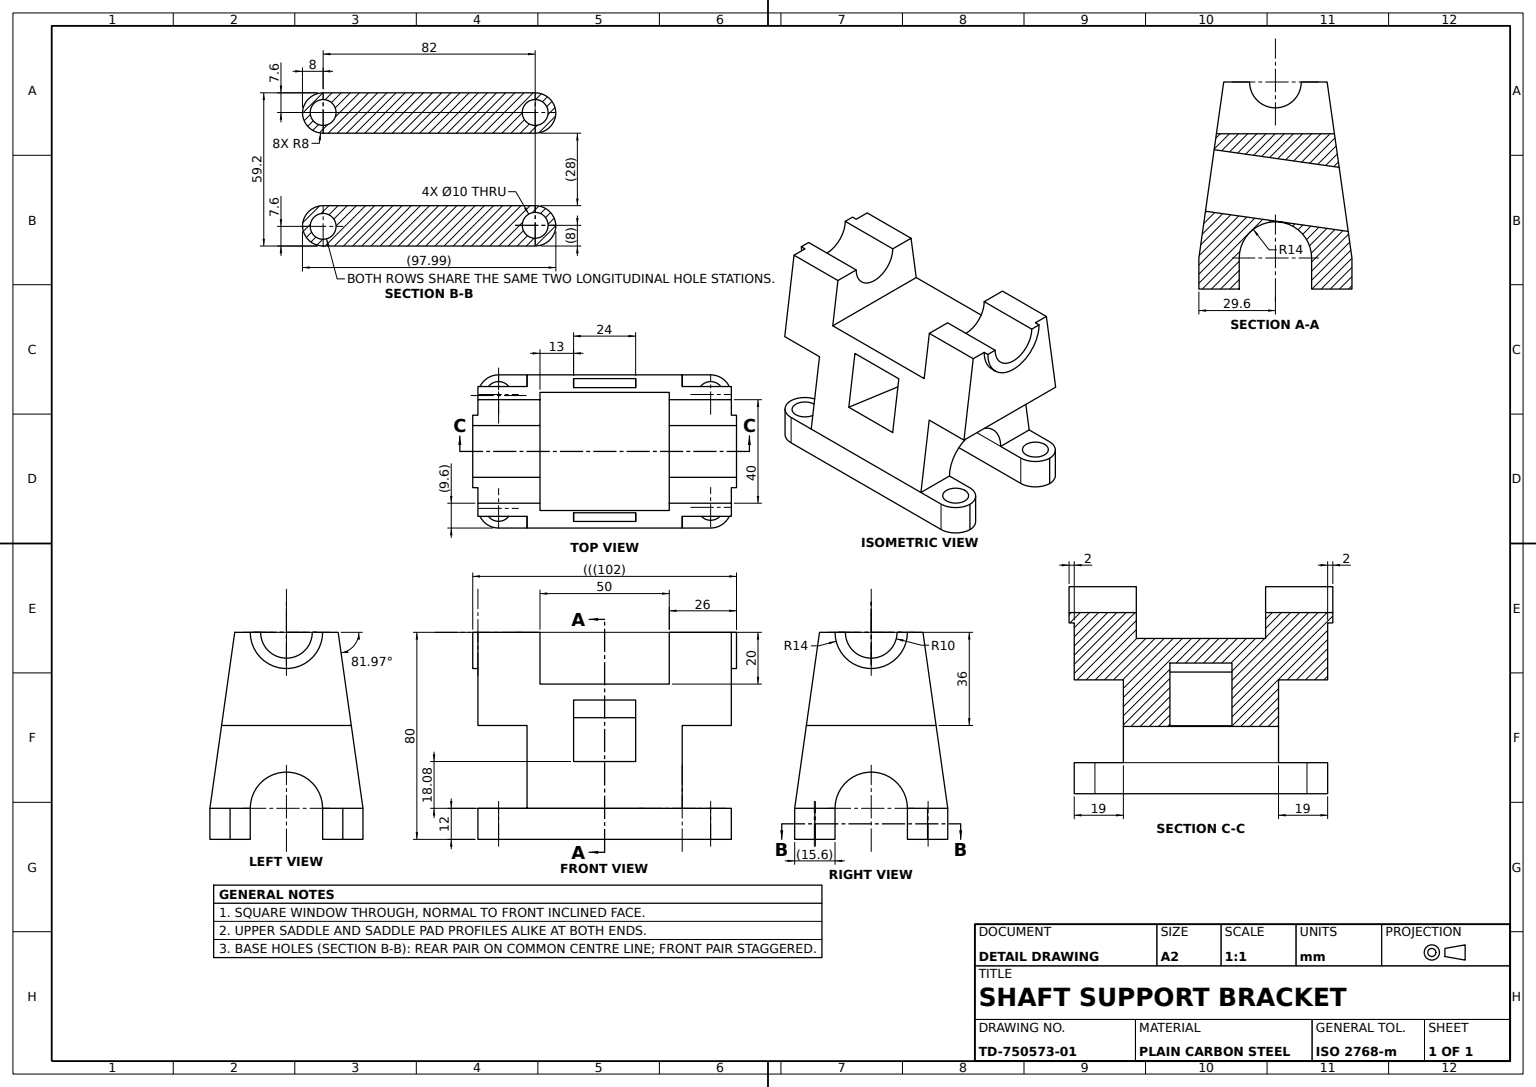
ISO-10303-21;
HEADER;
FILE_DESCRIPTION((''),'2;1');
FILE_NAME('','',(''),(''),'','','');
FILE_SCHEMA(('AUTOMOTIVE_DESIGN'));
ENDSEC;
DATA;
#1=APPLICATION_CONTEXT('');
#2=PRODUCT_CONTEXT('',#1,'mechanical');
#3=PRODUCT('','','',(#2));
#4=PRODUCT_DEFINITION_FORMATION('','',#3);
#5=PRODUCT_DEFINITION_CONTEXT('',#1,'design');
#6=PRODUCT_DEFINITION('','',#4,#5);
#7=PRODUCT_DEFINITION_SHAPE('','',#6);
#8=(LENGTH_UNIT()NAMED_UNIT(*)SI_UNIT(.MILLI.,.METRE.));
#9=(NAMED_UNIT(*)PLANE_ANGLE_UNIT()SI_UNIT($,.RADIAN.));
#10=(NAMED_UNIT(*)SI_UNIT($,.STERADIAN.)SOLID_ANGLE_UNIT());
#11=UNCERTAINTY_MEASURE_WITH_UNIT(LENGTH_MEASURE(1.E-05),#8,'distance_accuracy_value','');
#12=(GEOMETRIC_REPRESENTATION_CONTEXT(3)GLOBAL_UNCERTAINTY_ASSIGNED_CONTEXT((#11))GLOBAL_UNIT_ASSIGNED_CONTEXT((#8,#9,#10))REPRESENTATION_CONTEXT('',''));
#13=CARTESIAN_POINT('',(-49.,80.,-20.));
#14=VERTEX_POINT('',#13);
#15=CARTESIAN_POINT('',(-49.,80.,-14.));
#16=VERTEX_POINT('',#15);
#17=CARTESIAN_POINT('',(-49.,80.,20.));
#18=DIRECTION('',(0.,0.,1.));
#19=VECTOR('',#18,1000.);
#20=LINE('',#17,#19);
#21=EDGE_CURVE('',#14,#16,#20,.T.);
#22=ORIENTED_EDGE('',*,*,#21,.F.);
#23=CARTESIAN_POINT('',(-49.,44.,-25.081638));
#24=VERTEX_POINT('',#23);
#25=CARTESIAN_POINT('',(-49.,12.,-29.598649));
#26=DIRECTION('',(0.,0.990183858,0.139770985));
#27=VECTOR('',#26,1000.);
#28=LINE('',#25,#27);
#29=EDGE_CURVE('',#24,#14,#28,.T.);
#30=ORIENTED_EDGE('',*,*,#29,.F.);
#31=CARTESIAN_POINT('',(-49.,44.,25.081638));
#32=VERTEX_POINT('',#31);
#33=DIRECTION('',(0.,0.,-1.));
#34=VECTOR('',#33,1000.);
#35=LINE('',#23,#34);
#36=EDGE_CURVE('',#32,#24,#35,.T.);
#37=ORIENTED_EDGE('',*,*,#36,.F.);
#38=VERTEX_POINT('',#17);
#39=DIRECTION('',(0.,-0.990183858,0.139770985));
#40=VECTOR('',#39,1000.);
#41=LINE('',#17,#40);
#42=EDGE_CURVE('',#38,#32,#41,.T.);
#43=ORIENTED_EDGE('',*,*,#42,.F.);
#44=CARTESIAN_POINT('',(-49.,80.,14.));
#45=VERTEX_POINT('',#44);
#46=EDGE_CURVE('',#45,#38,#20,.T.);
#47=ORIENTED_EDGE('',*,*,#46,.F.);
#48=CARTESIAN_POINT('',(-49.,80.,0.));
#49=DIRECTION('',(-1.,0.,0.));
#50=AXIS2_PLACEMENT_3D('',#48,#49,#18);
#51=CIRCLE('',#50,14.);
#52=EDGE_CURVE('',#16,#45,#51,.T.);
#53=ORIENTED_EDGE('',*,*,#52,.F.);
#54=EDGE_LOOP('',(#22,#30,#37,#43,#47,#53));
#55=FACE_OUTER_BOUND('',#54,.T.);
#56=CARTESIAN_POINT('',(-49.,12.,29.598649));
#57=DIRECTION('',(1.,0.,0.));
#58=AXIS2_PLACEMENT_3D('',#56,#57,#33);
#59=PLANE('',#58);
#60=ADVANCED_FACE('',(#55),#59,.F.);
#61=CARTESIAN_POINT('',(-41.,0.,17.));
#62=VERTEX_POINT('',#61);
#63=CARTESIAN_POINT('',(-41.,12.,17.));
#64=VERTEX_POINT('',#63);
#65=CARTESIAN_POINT('',(-41.,-8.,17.));
#66=DIRECTION('',(0.,1.,0.));
#67=VECTOR('',#66,1000.);
#68=LINE('',#65,#67);
#69=EDGE_CURVE('',#62,#64,#68,.T.);
#70=ORIENTED_EDGE('',*,*,#69,.F.);
#71=CARTESIAN_POINT('',(-41.,0.,27.));
#72=VERTEX_POINT('',#71);
#73=CARTESIAN_POINT('',(-41.,0.,22.));
#74=DIRECTION('',(0.,-1.,0.));
#75=AXIS2_PLACEMENT_3D('',#73,#74,#33);
#76=CIRCLE('',#75,5.);
#77=EDGE_CURVE('',#62,#72,#76,.T.);
#78=ORIENTED_EDGE('',*,*,#77,.T.);
#79=CARTESIAN_POINT('',(-41.,12.,27.));
#80=VERTEX_POINT('',#79);
#81=CARTESIAN_POINT('',(-41.,-8.,27.));
#82=LINE('',#81,#67);
#83=EDGE_CURVE('',#72,#80,#82,.T.);
#84=ORIENTED_EDGE('',*,*,#83,.T.);
#85=CARTESIAN_POINT('',(-41.,12.,22.));
#86=AXIS2_PLACEMENT_3D('',#85,#66,#18);
#87=CIRCLE('',#86,5.);
#88=EDGE_CURVE('',#80,#64,#87,.T.);
#89=ORIENTED_EDGE('',*,*,#88,.T.);
#90=EDGE_LOOP('',(#70,#78,#84,#89));
#91=FACE_OUTER_BOUND('',#90,.T.);
#92=CARTESIAN_POINT('',(-41.,-8.,22.));
#93=AXIS2_PLACEMENT_3D('',#92,#66,#18);
#94=CYLINDRICAL_SURFACE('',#93,5.);
#95=ADVANCED_FACE('',(#91),#94,.F.);
#96=CARTESIAN_POINT('',(30.,44.,-25.081638));
#97=VERTEX_POINT('',#96);
#98=CARTESIAN_POINT('',(30.,44.,25.081638));
#99=VERTEX_POINT('',#98);
#100=LINE('',#98,#19);
#101=EDGE_CURVE('',#97,#99,#100,.T.);
#102=ORIENTED_EDGE('',*,*,#101,.T.);
#103=CARTESIAN_POINT('',(30.,12.,29.598649));
#104=VERTEX_POINT('',#103);
#105=LINE('',#103,#40);
#106=EDGE_CURVE('',#99,#104,#105,.T.);
#107=ORIENTED_EDGE('',*,*,#106,.T.);
#108=CARTESIAN_POINT('',(30.,12.,14.));
#109=VERTEX_POINT('',#108);
#110=LINE('',#108,#34);
#111=EDGE_CURVE('',#104,#109,#110,.T.);
#112=ORIENTED_EDGE('',*,*,#111,.T.);
#113=CARTESIAN_POINT('',(30.,12.,-14.));
#114=VERTEX_POINT('',#113);
#115=CARTESIAN_POINT('',(30.,12.,0.));
#116=AXIS2_PLACEMENT_3D('',#115,#49,#33);
#117=CIRCLE('',#116,14.);
#118=EDGE_CURVE('',#109,#114,#117,.T.);
#119=ORIENTED_EDGE('',*,*,#118,.T.);
#120=CARTESIAN_POINT('',(30.,12.,-29.598649));
#121=VERTEX_POINT('',#120);
#122=LINE('',#120,#34);
#123=EDGE_CURVE('',#114,#121,#122,.T.);
#124=ORIENTED_EDGE('',*,*,#123,.T.);
#125=LINE('',#96,#27);
#126=EDGE_CURVE('',#121,#97,#125,.T.);
#127=ORIENTED_EDGE('',*,*,#126,.T.);
#128=EDGE_LOOP('',(#102,#107,#112,#119,#124,#127));
#129=FACE_OUTER_BOUND('',#128,.T.);
#130=AXIS2_PLACEMENT_3D('',#115,#57,#33);
#131=PLANE('',#130);
#132=ADVANCED_FACE('',(#129),#131,.T.);
#133=CARTESIAN_POINT('',(-30.,44.,25.081638));
#134=VERTEX_POINT('',#133);
#135=CARTESIAN_POINT('',(-30.,44.,-25.081638));
#136=VERTEX_POINT('',#135);
#137=LINE('',#135,#34);
#138=EDGE_CURVE('',#134,#136,#137,.T.);
#139=ORIENTED_EDGE('',*,*,#138,.F.);
#140=VECTOR('',#49,1000.);
#141=LINE('',#133,#140);
#142=EDGE_CURVE('',#134,#32,#141,.T.);
#143=ORIENTED_EDGE('',*,*,#142,.T.);
#144=ORIENTED_EDGE('',*,*,#36,.T.);
#145=LINE('',#135,#140);
#146=EDGE_CURVE('',#136,#24,#145,.T.);
#147=ORIENTED_EDGE('',*,*,#146,.F.);
#148=EDGE_LOOP('',(#139,#143,#144,#147));
#149=FACE_OUTER_BOUND('',#148,.T.);
#150=AXIS2_PLACEMENT_3D('',#135,#66,#18);
#151=PLANE('',#150);
#152=ADVANCED_FACE('',(#149),#151,.F.);
#153=CARTESIAN_POINT('',(41.,0.,-17.));
#154=VERTEX_POINT('',#153);
#155=CARTESIAN_POINT('',(41.,0.,-27.));
#156=VERTEX_POINT('',#155);
#157=CARTESIAN_POINT('',(41.,0.,-22.));
#158=AXIS2_PLACEMENT_3D('',#157,#74,#33);
#159=CIRCLE('',#158,5.);
#160=EDGE_CURVE('',#154,#156,#159,.T.);
#161=ORIENTED_EDGE('',*,*,#160,.F.);
#162=EDGE_CURVE('',#156,#154,#159,.T.);
#163=ORIENTED_EDGE('',*,*,#162,.F.);
#164=EDGE_LOOP('',(#161,#163));
#165=FACE_BOUND('',#164,.T.);
#166=CARTESIAN_POINT('',(48.997483,0.,-21.799324));
#167=VERTEX_POINT('',#166);
#168=CARTESIAN_POINT('',(41.,0.,-14.));
#169=VERTEX_POINT('',#168);
#170=CIRCLE('',#158,8.);
#171=EDGE_CURVE('',#167,#169,#170,.T.);
#172=ORIENTED_EDGE('',*,*,#171,.T.);
#173=CARTESIAN_POINT('',(-41.,0.,-14.));
#174=VERTEX_POINT('',#173);
#175=CARTESIAN_POINT('',(-49.,0.,-14.));
#176=VECTOR('',#57,1000.);
#177=LINE('',#175,#176);
#178=EDGE_CURVE('',#174,#169,#177,.T.);
#179=ORIENTED_EDGE('',*,*,#178,.F.);
#180=CARTESIAN_POINT('',(-48.997483,0.,-21.799324));
#181=VERTEX_POINT('',#180);
#182=CARTESIAN_POINT('',(-41.,0.,-22.));
#183=AXIS2_PLACEMENT_3D('',#182,#74,#33);
#184=CIRCLE('',#183,8.);
#185=EDGE_CURVE('',#174,#181,#184,.T.);
#186=ORIENTED_EDGE('',*,*,#185,.T.);
#187=CARTESIAN_POINT('',(-41.,0.,-29.598649));
#188=VERTEX_POINT('',#187);
#189=CARTESIAN_POINT('',(-41.,0.,-21.598649));
#190=AXIS2_PLACEMENT_3D('',#189,#74,#33);
#191=CIRCLE('',#190,8.);
#192=EDGE_CURVE('',#181,#188,#191,.T.);
#193=ORIENTED_EDGE('',*,*,#192,.T.);
#194=CARTESIAN_POINT('',(41.,0.,-29.598649));
#195=VERTEX_POINT('',#194);
#196=CARTESIAN_POINT('',(-49.,0.,-29.598649));
#197=LINE('',#196,#140);
#198=EDGE_CURVE('',#195,#188,#197,.T.);
#199=ORIENTED_EDGE('',*,*,#198,.F.);
#200=CARTESIAN_POINT('',(41.,0.,-21.598649));
#201=AXIS2_PLACEMENT_3D('',#200,#74,#33);
#202=CIRCLE('',#201,8.);
#203=EDGE_CURVE('',#195,#167,#202,.T.);
#204=ORIENTED_EDGE('',*,*,#203,.T.);
#205=EDGE_LOOP('',(#172,#179,#186,#193,#199,#204));
#206=FACE_OUTER_BOUND('',#205,.T.);
#207=CARTESIAN_POINT('',(-41.,0.,-27.));
#208=VERTEX_POINT('',#207);
#209=CARTESIAN_POINT('',(-41.,0.,-17.));
#210=VERTEX_POINT('',#209);
#211=CIRCLE('',#183,5.);
#212=EDGE_CURVE('',#208,#210,#211,.T.);
#213=ORIENTED_EDGE('',*,*,#212,.F.);
#214=EDGE_CURVE('',#210,#208,#211,.T.);
#215=ORIENTED_EDGE('',*,*,#214,.F.);
#216=EDGE_LOOP('',(#213,#215));
#217=FACE_BOUND('',#216,.T.);
#218=CARTESIAN_POINT('',(0.,0.,0.));
#219=AXIS2_PLACEMENT_3D('',#218,#74,#33);
#220=PLANE('',#219);
#221=ADVANCED_FACE('',(#165,#206,#217),#220,.T.);
#222=CARTESIAN_POINT('',(-51.,80.,-10.));
#223=VERTEX_POINT('',#222);
#224=CARTESIAN_POINT('',(-51.,80.,10.));
#225=VERTEX_POINT('',#224);
#226=CARTESIAN_POINT('',(-51.,80.,0.));
#227=AXIS2_PLACEMENT_3D('',#226,#49,#18);
#228=CIRCLE('',#227,10.);
#229=EDGE_CURVE('',#223,#225,#228,.T.);
#230=ORIENTED_EDGE('',*,*,#229,.F.);
#231=CARTESIAN_POINT('',(-51.,80.,-14.));
#232=VERTEX_POINT('',#231);
#233=LINE('',#231,#34);
#234=EDGE_CURVE('',#223,#232,#233,.T.);
#235=ORIENTED_EDGE('',*,*,#234,.T.);
#236=CARTESIAN_POINT('',(-51.,80.,14.));
#237=VERTEX_POINT('',#236);
#238=CIRCLE('',#227,14.);
#239=EDGE_CURVE('',#232,#237,#238,.T.);
#240=ORIENTED_EDGE('',*,*,#239,.T.);
#241=EDGE_CURVE('',#237,#225,#233,.T.);
#242=ORIENTED_EDGE('',*,*,#241,.T.);
#243=EDGE_LOOP('',(#230,#235,#240,#242));
#244=FACE_OUTER_BOUND('',#243,.T.);
#245=PLANE('',#227);
#246=ADVANCED_FACE('',(#244),#245,.T.);
#247=CARTESIAN_POINT('',(41.,12.,-17.));
#248=VERTEX_POINT('',#247);
#249=CARTESIAN_POINT('',(41.,-8.,-17.));
#250=LINE('',#249,#67);
#251=EDGE_CURVE('',#154,#248,#250,.T.);
#252=ORIENTED_EDGE('',*,*,#251,.T.);
#253=CARTESIAN_POINT('',(41.,12.,-27.));
#254=VERTEX_POINT('',#253);
#255=CARTESIAN_POINT('',(41.,12.,-22.));
#256=AXIS2_PLACEMENT_3D('',#255,#66,#18);
#257=CIRCLE('',#256,5.);
#258=EDGE_CURVE('',#248,#254,#257,.T.);
#259=ORIENTED_EDGE('',*,*,#258,.T.);
#260=CARTESIAN_POINT('',(41.,-8.,-27.));
#261=LINE('',#260,#67);
#262=EDGE_CURVE('',#156,#254,#261,.T.);
#263=ORIENTED_EDGE('',*,*,#262,.F.);
#264=ORIENTED_EDGE('',*,*,#162,.T.);
#265=EDGE_LOOP('',(#252,#259,#263,#264));
#266=FACE_OUTER_BOUND('',#265,.T.);
#267=CARTESIAN_POINT('',(41.,-8.,-22.));
#268=AXIS2_PLACEMENT_3D('',#267,#66,#18);
#269=CYLINDRICAL_SURFACE('',#268,5.);
#270=ADVANCED_FACE('',(#266),#269,.F.);
#271=ORIENTED_EDGE('',*,*,#212,.T.);
#272=CARTESIAN_POINT('',(-41.,12.,-17.));
#273=VERTEX_POINT('',#272);
#274=CARTESIAN_POINT('',(-41.,-8.,-17.));
#275=LINE('',#274,#67);
#276=EDGE_CURVE('',#210,#273,#275,.T.);
#277=ORIENTED_EDGE('',*,*,#276,.T.);
#278=CARTESIAN_POINT('',(-41.,12.,-27.));
#279=VERTEX_POINT('',#278);
#280=CARTESIAN_POINT('',(-41.,12.,-22.));
#281=AXIS2_PLACEMENT_3D('',#280,#66,#18);
#282=CIRCLE('',#281,5.);
#283=EDGE_CURVE('',#273,#279,#282,.T.);
#284=ORIENTED_EDGE('',*,*,#283,.T.);
#285=CARTESIAN_POINT('',(-41.,-8.,-27.));
#286=LINE('',#285,#67);
#287=EDGE_CURVE('',#208,#279,#286,.T.);
#288=ORIENTED_EDGE('',*,*,#287,.F.);
#289=EDGE_LOOP('',(#271,#277,#284,#288));
#290=FACE_OUTER_BOUND('',#289,.T.);
#291=CARTESIAN_POINT('',(-41.,-8.,-22.));
#292=AXIS2_PLACEMENT_3D('',#291,#66,#18);
#293=CYLINDRICAL_SURFACE('',#292,5.);
#294=ADVANCED_FACE('',(#290),#293,.F.);
#295=CARTESIAN_POINT('',(25.,80.,20.));
#296=VERTEX_POINT('',#295);
#297=CARTESIAN_POINT('',(25.,80.,10.));
#298=VERTEX_POINT('',#297);
#299=CARTESIAN_POINT('',(25.,80.,26.));
#300=LINE('',#299,#34);
#301=EDGE_CURVE('',#296,#298,#300,.T.);
#302=ORIENTED_EDGE('',*,*,#301,.F.);
#303=CARTESIAN_POINT('',(49.,80.,20.));
#304=VERTEX_POINT('',#303);
#305=LINE('',#17,#176);
#306=EDGE_CURVE('',#296,#304,#305,.T.);
#307=ORIENTED_EDGE('',*,*,#306,.T.);
#308=CARTESIAN_POINT('',(49.,80.,14.));
#309=VERTEX_POINT('',#308);
#310=LINE('',#303,#19);
#311=EDGE_CURVE('',#309,#304,#310,.T.);
#312=ORIENTED_EDGE('',*,*,#311,.F.);
#313=CARTESIAN_POINT('',(51.,80.,14.));
#314=VERTEX_POINT('',#313);
#315=CARTESIAN_POINT('',(25.,80.,14.));
#316=LINE('',#315,#176);
#317=EDGE_CURVE('',#309,#314,#316,.T.);
#318=ORIENTED_EDGE('',*,*,#317,.T.);
#319=CARTESIAN_POINT('',(51.,80.,10.));
#320=VERTEX_POINT('',#319);
#321=CARTESIAN_POINT('',(51.,80.,0.));
#322=LINE('',#321,#34);
#323=EDGE_CURVE('',#314,#320,#322,.T.);
#324=ORIENTED_EDGE('',*,*,#323,.T.);
#325=LINE('',#297,#176);
#326=EDGE_CURVE('',#298,#320,#325,.T.);
#327=ORIENTED_EDGE('',*,*,#326,.F.);
#328=EDGE_LOOP('',(#302,#307,#312,#318,#324,#327));
#329=FACE_OUTER_BOUND('',#328,.T.);
#330=AXIS2_PLACEMENT_3D('',#17,#66,#18);
#331=PLANE('',#330);
#332=ADVANCED_FACE('',(#329),#331,.T.);
#333=CARTESIAN_POINT('',(-30.,12.,-14.));
#334=VERTEX_POINT('',#333);
#335=CARTESIAN_POINT('',(-30.,12.,14.));
#336=VERTEX_POINT('',#335);
#337=CARTESIAN_POINT('',(-30.,12.,0.));
#338=AXIS2_PLACEMENT_3D('',#337,#57,#18);
#339=CIRCLE('',#338,14.);
#340=EDGE_CURVE('',#334,#336,#339,.T.);
#341=ORIENTED_EDGE('',*,*,#340,.T.);
#342=CARTESIAN_POINT('',(-30.,12.,29.598649));
#343=VERTEX_POINT('',#342);
#344=LINE('',#342,#19);
#345=EDGE_CURVE('',#336,#343,#344,.T.);
#346=ORIENTED_EDGE('',*,*,#345,.T.);
#347=DIRECTION('',(0.,0.990183858,-0.139770985));
#348=VECTOR('',#347,1000.);
#349=LINE('',#133,#348);
#350=EDGE_CURVE('',#343,#134,#349,.T.);
#351=ORIENTED_EDGE('',*,*,#350,.T.);
#352=ORIENTED_EDGE('',*,*,#138,.T.);
#353=CARTESIAN_POINT('',(-30.,12.,-29.598649));
#354=VERTEX_POINT('',#353);
#355=DIRECTION('',(0.,-0.990183858,-0.139770985));
#356=VECTOR('',#355,1000.);
#357=LINE('',#353,#356);
#358=EDGE_CURVE('',#136,#354,#357,.T.);
#359=ORIENTED_EDGE('',*,*,#358,.T.);
#360=LINE('',#333,#19);
#361=EDGE_CURVE('',#354,#334,#360,.T.);
#362=ORIENTED_EDGE('',*,*,#361,.T.);
#363=EDGE_LOOP('',(#341,#346,#351,#352,#359,#362));
#364=FACE_OUTER_BOUND('',#363,.T.);
#365=AXIS2_PLACEMENT_3D('',#337,#49,#18);
#366=PLANE('',#365);
#367=ADVANCED_FACE('',(#364),#366,.T.);
#368=ORIENTED_EDGE('',*,*,#214,.T.);
#369=ORIENTED_EDGE('',*,*,#287,.T.);
#370=EDGE_CURVE('',#279,#273,#282,.T.);
#371=ORIENTED_EDGE('',*,*,#370,.T.);
#372=ORIENTED_EDGE('',*,*,#276,.F.);
#373=EDGE_LOOP('',(#368,#369,#371,#372));
#374=FACE_OUTER_BOUND('',#373,.T.);
#375=ADVANCED_FACE('',(#374),#293,.F.);
#376=CARTESIAN_POINT('',(-48.997483,0.,21.799324));
#377=VERTEX_POINT('',#376);
#378=CARTESIAN_POINT('',(-41.,0.,14.));
#379=VERTEX_POINT('',#378);
#380=CIRCLE('',#75,8.);
#381=EDGE_CURVE('',#377,#379,#380,.T.);
#382=ORIENTED_EDGE('',*,*,#381,.F.);
#383=CARTESIAN_POINT('',(-48.997483,12.,21.799324));
#384=VERTEX_POINT('',#383);
#385=CARTESIAN_POINT('',(-48.997483,6.,21.799324));
#386=VECTOR('',#74,1000.);
#387=LINE('',#385,#386);
#388=EDGE_CURVE('',#384,#377,#387,.T.);
#389=ORIENTED_EDGE('',*,*,#388,.F.);
#390=CARTESIAN_POINT('',(-41.,12.,14.));
#391=VERTEX_POINT('',#390);
#392=AXIS2_PLACEMENT_3D('',#85,#66,#33);
#393=CIRCLE('',#392,8.);
#394=EDGE_CURVE('',#391,#384,#393,.T.);
#395=ORIENTED_EDGE('',*,*,#394,.F.);
#396=LINE('',#390,#67);
#397=EDGE_CURVE('',#379,#391,#396,.T.);
#398=ORIENTED_EDGE('',*,*,#397,.F.);
#399=EDGE_LOOP('',(#382,#389,#395,#398));
#400=FACE_OUTER_BOUND('',#399,.T.);
#401=AXIS2_PLACEMENT_3D('',#85,#74,#33);
#402=CYLINDRICAL_SURFACE('',#401,8.);
#403=ADVANCED_FACE('',(#400),#402,.T.);
#404=ORIENTED_EDGE('',*,*,#340,.F.);
#405=CARTESIAN_POINT('',(-49.,12.,-14.));
#406=LINE('',#405,#176);
#407=EDGE_CURVE('',#334,#114,#406,.T.);
#408=ORIENTED_EDGE('',*,*,#407,.T.);
#409=ORIENTED_EDGE('',*,*,#118,.F.);
#410=CARTESIAN_POINT('',(-49.,12.,14.));
#411=LINE('',#410,#176);
#412=EDGE_CURVE('',#336,#109,#411,.T.);
#413=ORIENTED_EDGE('',*,*,#412,.F.);
#414=EDGE_LOOP('',(#404,#408,#409,#413));
#415=FACE_OUTER_BOUND('',#414,.T.);
#416=CARTESIAN_POINT('',(-49.,12.,0.));
#417=AXIS2_PLACEMENT_3D('',#416,#57,#33);
#418=CYLINDRICAL_SURFACE('',#417,14.);
#419=ADVANCED_FACE('',(#415),#418,.F.);
#420=CARTESIAN_POINT('',(41.,12.,26.598649));
#421=VERTEX_POINT('',#420);
#422=CARTESIAN_POINT('',(41.,12.,16.598649));
#423=VERTEX_POINT('',#422);
#424=CARTESIAN_POINT('',(41.,12.,21.598649));
#425=AXIS2_PLACEMENT_3D('',#424,#66,#18);
#426=CIRCLE('',#425,5.);
#427=EDGE_CURVE('',#421,#423,#426,.T.);
#428=ORIENTED_EDGE('',*,*,#427,.T.);
#429=CARTESIAN_POINT('',(41.,0.,16.598649));
#430=VERTEX_POINT('',#429);
#431=CARTESIAN_POINT('',(41.,-8.,16.598649));
#432=LINE('',#431,#67);
#433=EDGE_CURVE('',#430,#423,#432,.T.);
#434=ORIENTED_EDGE('',*,*,#433,.F.);
#435=CARTESIAN_POINT('',(41.,0.,26.598649));
#436=VERTEX_POINT('',#435);
#437=CARTESIAN_POINT('',(41.,0.,21.598649));
#438=AXIS2_PLACEMENT_3D('',#437,#74,#33);
#439=CIRCLE('',#438,5.);
#440=EDGE_CURVE('',#430,#436,#439,.T.);
#441=ORIENTED_EDGE('',*,*,#440,.T.);
#442=CARTESIAN_POINT('',(41.,-8.,26.598649));
#443=LINE('',#442,#67);
#444=EDGE_CURVE('',#436,#421,#443,.T.);
#445=ORIENTED_EDGE('',*,*,#444,.T.);
#446=EDGE_LOOP('',(#428,#434,#441,#445));
#447=FACE_OUTER_BOUND('',#446,.T.);
#448=CARTESIAN_POINT('',(41.,-8.,21.598649));
#449=AXIS2_PLACEMENT_3D('',#448,#66,#18);
#450=CYLINDRICAL_SURFACE('',#449,5.);
#451=ADVANCED_FACE('',(#447),#450,.F.);
#452=CARTESIAN_POINT('',(49.,80.,-14.));
#453=VERTEX_POINT('',#452);
#454=CARTESIAN_POINT('',(49.,80.,0.));
#455=AXIS2_PLACEMENT_3D('',#454,#49,#18);
#456=CIRCLE('',#455,14.);
#457=EDGE_CURVE('',#453,#309,#456,.T.);
#458=ORIENTED_EDGE('',*,*,#457,.F.);
#459=CARTESIAN_POINT('',(51.,80.,-14.));
#460=VERTEX_POINT('',#459);
#461=CARTESIAN_POINT('',(25.,80.,-14.));
#462=LINE('',#461,#176);
#463=EDGE_CURVE('',#453,#460,#462,.T.);
#464=ORIENTED_EDGE('',*,*,#463,.T.);
#465=AXIS2_PLACEMENT_3D('',#321,#57,#33);
#466=CIRCLE('',#465,14.);
#467=EDGE_CURVE('',#314,#460,#466,.T.);
#468=ORIENTED_EDGE('',*,*,#467,.F.);
#469=ORIENTED_EDGE('',*,*,#317,.F.);
#470=EDGE_LOOP('',(#458,#464,#468,#469));
#471=FACE_OUTER_BOUND('',#470,.T.);
#472=CARTESIAN_POINT('',(25.,80.,0.));
#473=AXIS2_PLACEMENT_3D('',#472,#57,#33);
#474=CYLINDRICAL_SURFACE('',#473,14.);
#475=ADVANCED_FACE('',(#471),#474,.T.);
#476=CARTESIAN_POINT('',(41.,12.,-14.));
#477=VERTEX_POINT('',#476);
#478=LINE('',#168,#67);
#479=EDGE_CURVE('',#169,#477,#478,.T.);
#480=ORIENTED_EDGE('',*,*,#479,.F.);
#481=ORIENTED_EDGE('',*,*,#171,.F.);
#482=CARTESIAN_POINT('',(48.997483,12.,-21.799324));
#483=VERTEX_POINT('',#482);
#484=CARTESIAN_POINT('',(48.997483,6.,-21.799324));
#485=LINE('',#484,#386);
#486=EDGE_CURVE('',#483,#167,#485,.T.);
#487=ORIENTED_EDGE('',*,*,#486,.F.);
#488=AXIS2_PLACEMENT_3D('',#255,#66,#33);
#489=CIRCLE('',#488,8.);
#490=EDGE_CURVE('',#477,#483,#489,.T.);
#491=ORIENTED_EDGE('',*,*,#490,.F.);
#492=EDGE_LOOP('',(#480,#481,#487,#491));
#493=FACE_OUTER_BOUND('',#492,.T.);
#494=AXIS2_PLACEMENT_3D('',#157,#66,#18);
#495=CYLINDRICAL_SURFACE('',#494,8.);
#496=ADVANCED_FACE('',(#493),#495,.T.);
#497=CARTESIAN_POINT('',(-25.,60.,22.823132));
#498=VERTEX_POINT('',#497);
#499=CARTESIAN_POINT('',(25.,60.,22.823132));
#500=VERTEX_POINT('',#499);
#501=CARTESIAN_POINT('',(-49.,60.,22.823132));
#502=LINE('',#501,#176);
#503=EDGE_CURVE('',#498,#500,#502,.T.);
#504=ORIENTED_EDGE('',*,*,#503,.T.);
#505=CARTESIAN_POINT('',(25.,60.,-22.823132));
#506=VERTEX_POINT('',#505);
#507=CARTESIAN_POINT('',(25.,60.,26.));
#508=LINE('',#507,#34);
#509=EDGE_CURVE('',#500,#506,#508,.T.);
#510=ORIENTED_EDGE('',*,*,#509,.T.);
#511=CARTESIAN_POINT('',(-25.,60.,-22.823132));
#512=VERTEX_POINT('',#511);
#513=CARTESIAN_POINT('',(-49.,60.,-22.823132));
#514=LINE('',#513,#140);
#515=EDGE_CURVE('',#506,#512,#514,.T.);
#516=ORIENTED_EDGE('',*,*,#515,.T.);
#517=CARTESIAN_POINT('',(-25.,60.,26.));
#518=LINE('',#517,#19);
#519=EDGE_CURVE('',#512,#498,#518,.T.);
#520=ORIENTED_EDGE('',*,*,#519,.T.);
#521=EDGE_LOOP('',(#504,#510,#516,#520));
#522=FACE_OUTER_BOUND('',#521,.T.);
#523=CARTESIAN_POINT('',(0.,60.,0.));
#524=AXIS2_PLACEMENT_3D('',#523,#74,#33);
#525=PLANE('',#524);
#526=ADVANCED_FACE('',(#522),#525,.F.);
#527=ORIENTED_EDGE('',*,*,#69,.T.);
#528=EDGE_CURVE('',#64,#80,#87,.T.);
#529=ORIENTED_EDGE('',*,*,#528,.T.);
#530=ORIENTED_EDGE('',*,*,#83,.F.);
#531=EDGE_CURVE('',#72,#62,#76,.T.);
#532=ORIENTED_EDGE('',*,*,#531,.T.);
#533=EDGE_LOOP('',(#527,#529,#530,#532));
#534=FACE_OUTER_BOUND('',#533,.T.);
#535=ADVANCED_FACE('',(#534),#94,.F.);
#536=ORIENTED_EDGE('',*,*,#479,.T.);
#537=LINE('',#113,#176);
#538=EDGE_CURVE('',#114,#477,#537,.T.);
#539=ORIENTED_EDGE('',*,*,#538,.F.);
#540=ORIENTED_EDGE('',*,*,#407,.F.);
#541=CARTESIAN_POINT('',(-41.,12.,-14.));
#542=VERTEX_POINT('',#541);
#543=EDGE_CURVE('',#542,#334,#406,.T.);
#544=ORIENTED_EDGE('',*,*,#543,.F.);
#545=LINE('',#173,#386);
#546=EDGE_CURVE('',#542,#174,#545,.T.);
#547=ORIENTED_EDGE('',*,*,#546,.T.);
#548=ORIENTED_EDGE('',*,*,#178,.T.);
#549=EDGE_LOOP('',(#536,#539,#540,#544,#547,#548));
#550=FACE_OUTER_BOUND('',#549,.T.);
#551=AXIS2_PLACEMENT_3D('',#175,#33,#66);
#552=PLANE('',#551);
#553=ADVANCED_FACE('',(#550),#552,.F.);
#554=ORIENTED_EDGE('',*,*,#323,.F.);
#555=ORIENTED_EDGE('',*,*,#467,.T.);
#556=CARTESIAN_POINT('',(51.,80.,-10.));
#557=VERTEX_POINT('',#556);
#558=EDGE_CURVE('',#557,#460,#322,.T.);
#559=ORIENTED_EDGE('',*,*,#558,.F.);
#560=CIRCLE('',#465,10.);
#561=EDGE_CURVE('',#320,#557,#560,.T.);
#562=ORIENTED_EDGE('',*,*,#561,.F.);
#563=EDGE_LOOP('',(#554,#555,#559,#562));
#564=FACE_OUTER_BOUND('',#563,.T.);
#565=CARTESIAN_POINT('',(51.,0.,0.));
#566=AXIS2_PLACEMENT_3D('',#565,#57,#33);
#567=PLANE('',#566);
#568=ADVANCED_FACE('',(#564),#567,.T.);
#569=ORIENTED_EDGE('',*,*,#440,.F.);
#570=EDGE_CURVE('',#436,#430,#439,.T.);
#571=ORIENTED_EDGE('',*,*,#570,.F.);
#572=EDGE_LOOP('',(#569,#571));
#573=FACE_BOUND('',#572,.T.);
#574=ORIENTED_EDGE('',*,*,#531,.F.);
#575=ORIENTED_EDGE('',*,*,#77,.F.);
#576=EDGE_LOOP('',(#574,#575));
#577=FACE_BOUND('',#576,.T.);
#578=CARTESIAN_POINT('',(41.,0.,14.));
#579=VERTEX_POINT('',#578);
#580=CARTESIAN_POINT('',(48.997483,0.,21.799324));
#581=VERTEX_POINT('',#580);
#582=CARTESIAN_POINT('',(41.,0.,22.));
#583=AXIS2_PLACEMENT_3D('',#582,#74,#33);
#584=CIRCLE('',#583,8.);
#585=EDGE_CURVE('',#579,#581,#584,.T.);
#586=ORIENTED_EDGE('',*,*,#585,.T.);
#587=CARTESIAN_POINT('',(41.,0.,29.598649));
#588=VERTEX_POINT('',#587);
#589=CIRCLE('',#438,8.);
#590=EDGE_CURVE('',#581,#588,#589,.T.);
#591=ORIENTED_EDGE('',*,*,#590,.T.);
#592=CARTESIAN_POINT('',(-41.,0.,29.598649));
#593=VERTEX_POINT('',#592);
#594=CARTESIAN_POINT('',(-49.,0.,29.598649));
#595=LINE('',#594,#176);
#596=EDGE_CURVE('',#593,#588,#595,.T.);
#597=ORIENTED_EDGE('',*,*,#596,.F.);
#598=CARTESIAN_POINT('',(-41.,0.,21.598649));
#599=AXIS2_PLACEMENT_3D('',#598,#74,#33);
#600=CIRCLE('',#599,8.);
#601=EDGE_CURVE('',#593,#377,#600,.T.);
#602=ORIENTED_EDGE('',*,*,#601,.T.);
#603=ORIENTED_EDGE('',*,*,#381,.T.);
#604=CARTESIAN_POINT('',(-49.,0.,14.));
#605=LINE('',#604,#176);
#606=EDGE_CURVE('',#379,#579,#605,.T.);
#607=ORIENTED_EDGE('',*,*,#606,.T.);
#608=EDGE_LOOP('',(#586,#591,#597,#602,#603,#607));
#609=FACE_OUTER_BOUND('',#608,.T.);
#610=ADVANCED_FACE('',(#573,#577,#609),#220,.T.);
#611=ORIENTED_EDGE('',*,*,#370,.F.);
#612=ORIENTED_EDGE('',*,*,#283,.F.);
#613=EDGE_LOOP('',(#611,#612));
#614=FACE_BOUND('',#613,.T.);
#615=CARTESIAN_POINT('',(-41.,12.,-29.598649));
#616=VERTEX_POINT('',#615);
#617=CARTESIAN_POINT('',(-48.997483,12.,-21.799324));
#618=VERTEX_POINT('',#617);
#619=CARTESIAN_POINT('',(-41.,12.,-21.598649));
#620=AXIS2_PLACEMENT_3D('',#619,#66,#33);
#621=CIRCLE('',#620,8.);
#622=EDGE_CURVE('',#616,#618,#621,.T.);
#623=ORIENTED_EDGE('',*,*,#622,.T.);
#624=AXIS2_PLACEMENT_3D('',#280,#66,#33);
#625=CIRCLE('',#624,8.);
#626=EDGE_CURVE('',#618,#542,#625,.T.);
#627=ORIENTED_EDGE('',*,*,#626,.T.);
#628=ORIENTED_EDGE('',*,*,#543,.T.);
#629=ORIENTED_EDGE('',*,*,#361,.F.);
#630=LINE('',#353,#140);
#631=EDGE_CURVE('',#354,#616,#630,.T.);
#632=ORIENTED_EDGE('',*,*,#631,.T.);
#633=EDGE_LOOP('',(#623,#627,#628,#629,#632));
#634=FACE_OUTER_BOUND('',#633,.T.);
#635=AXIS2_PLACEMENT_3D('',#333,#74,#33);
#636=PLANE('',#635);
#637=ADVANCED_FACE('',(#614,#634),#636,.F.);
#638=CARTESIAN_POINT('',(12.,30.075634,27.047154));
#639=VERTEX_POINT('',#638);
#640=CARTESIAN_POINT('',(12.,53.840047,23.69265));
#641=VERTEX_POINT('',#640);
#642=LINE('',#640,#348);
#643=EDGE_CURVE('',#639,#641,#642,.T.);
#644=ORIENTED_EDGE('',*,*,#643,.F.);
#645=CARTESIAN_POINT('',(-12.,30.075634,27.047154));
#646=VERTEX_POINT('',#645);
#647=LINE('',#645,#176);
#648=EDGE_CURVE('',#646,#639,#647,.T.);
#649=ORIENTED_EDGE('',*,*,#648,.F.);
#650=CARTESIAN_POINT('',(-12.,53.840047,23.69265));
#651=VERTEX_POINT('',#650);
#652=LINE('',#650,#40);
#653=EDGE_CURVE('',#651,#646,#652,.T.);
#654=ORIENTED_EDGE('',*,*,#653,.F.);
#655=LINE('',#650,#140);
#656=EDGE_CURVE('',#641,#651,#655,.T.);
#657=ORIENTED_EDGE('',*,*,#656,.F.);
#658=EDGE_LOOP('',(#644,#649,#654,#657));
#659=FACE_BOUND('',#658,.T.);
#660=CARTESIAN_POINT('',(-25.,80.,20.));
#661=VERTEX_POINT('',#660);
#662=EDGE_CURVE('',#38,#661,#305,.T.);
#663=ORIENTED_EDGE('',*,*,#662,.F.);
#664=ORIENTED_EDGE('',*,*,#42,.T.);
#665=ORIENTED_EDGE('',*,*,#142,.F.);
#666=ORIENTED_EDGE('',*,*,#350,.F.);
#667=LINE('',#56,#176);
#668=EDGE_CURVE('',#343,#104,#667,.T.);
#669=ORIENTED_EDGE('',*,*,#668,.T.);
#670=ORIENTED_EDGE('',*,*,#106,.F.);
#671=CARTESIAN_POINT('',(49.,44.,25.081638));
#672=VERTEX_POINT('',#671);
#673=LINE('',#98,#176);
#674=EDGE_CURVE('',#99,#672,#673,.T.);
#675=ORIENTED_EDGE('',*,*,#674,.T.);
#676=LINE('',#303,#40);
#677=EDGE_CURVE('',#304,#672,#676,.T.);
#678=ORIENTED_EDGE('',*,*,#677,.F.);
#679=ORIENTED_EDGE('',*,*,#306,.F.);
#680=LINE('',#295,#348);
#681=EDGE_CURVE('',#500,#296,#680,.T.);
#682=ORIENTED_EDGE('',*,*,#681,.F.);
#683=ORIENTED_EDGE('',*,*,#503,.F.);
#684=LINE('',#660,#40);
#685=EDGE_CURVE('',#661,#498,#684,.T.);
#686=ORIENTED_EDGE('',*,*,#685,.F.);
#687=EDGE_LOOP('',(#663,#664,#665,#666,#669,#670,#675,#678,#679,#682,#683,#686));
#688=FACE_OUTER_BOUND('',#687,.T.);
#689=DIRECTION('',(0.,0.139770985,0.990183858));
#690=AXIS2_PLACEMENT_3D('',#17,#689,#39);
#691=PLANE('',#690);
#692=ADVANCED_FACE('',(#659,#688),#691,.T.);
#693=CARTESIAN_POINT('',(41.,12.,-29.598649));
#694=VERTEX_POINT('',#693);
#695=LINE('',#693,#386);
#696=EDGE_CURVE('',#694,#195,#695,.T.);
#697=ORIENTED_EDGE('',*,*,#696,.F.);
#698=CARTESIAN_POINT('',(41.,12.,-21.598649));
#699=AXIS2_PLACEMENT_3D('',#698,#66,#33);
#700=CIRCLE('',#699,8.);
#701=EDGE_CURVE('',#483,#694,#700,.T.);
#702=ORIENTED_EDGE('',*,*,#701,.F.);
#703=ORIENTED_EDGE('',*,*,#486,.T.);
#704=ORIENTED_EDGE('',*,*,#203,.F.);
#705=EDGE_LOOP('',(#697,#702,#703,#704));
#706=FACE_OUTER_BOUND('',#705,.T.);
#707=AXIS2_PLACEMENT_3D('',#698,#74,#33);
#708=CYLINDRICAL_SURFACE('',#707,8.);
#709=ADVANCED_FACE('',(#706),#708,.T.);
#710=ORIENTED_EDGE('',*,*,#457,.T.);
#711=ORIENTED_EDGE('',*,*,#311,.T.);
#712=ORIENTED_EDGE('',*,*,#677,.T.);
#713=CARTESIAN_POINT('',(49.,44.,-25.081638));
#714=VERTEX_POINT('',#713);
#715=LINE('',#671,#19);
#716=EDGE_CURVE('',#714,#672,#715,.T.);
#717=ORIENTED_EDGE('',*,*,#716,.F.);
#718=CARTESIAN_POINT('',(49.,80.,-20.));
#719=VERTEX_POINT('',#718);
#720=CARTESIAN_POINT('',(49.,12.,-29.598649));
#721=LINE('',#720,#27);
#722=EDGE_CURVE('',#714,#719,#721,.T.);
#723=ORIENTED_EDGE('',*,*,#722,.T.);
#724=EDGE_CURVE('',#719,#453,#310,.T.);
#725=ORIENTED_EDGE('',*,*,#724,.T.);
#726=EDGE_LOOP('',(#710,#711,#712,#717,#723,#725));
#727=FACE_OUTER_BOUND('',#726,.T.);
#728=CARTESIAN_POINT('',(49.,12.,29.598649));
#729=AXIS2_PLACEMENT_3D('',#728,#49,#18);
#730=PLANE('',#729);
#731=ADVANCED_FACE('',(#727),#730,.F.);
#732=ORIENTED_EDGE('',*,*,#653,.T.);
#733=CARTESIAN_POINT('',(-12.,22.284628,-28.146905));
#734=VERTEX_POINT('',#733);
#735=CARTESIAN_POINT('',(-12.,21.648358,-32.654457));
#736=VECTOR('',#689,1000.);
#737=LINE('',#735,#736);
#738=EDGE_CURVE('',#734,#646,#737,.T.);
#739=ORIENTED_EDGE('',*,*,#738,.F.);
#740=CARTESIAN_POINT('',(-12.,47.015315,-24.656006));
#741=VERTEX_POINT('',#740);
#742=CARTESIAN_POINT('',(-12.,12.,-29.598649));
#743=LINE('',#742,#27);
#744=EDGE_CURVE('',#734,#741,#743,.T.);
#745=ORIENTED_EDGE('',*,*,#744,.T.);
#746=CARTESIAN_POINT('',(-12.,45.41277,-36.008961));
#747=LINE('',#746,#736);
#748=EDGE_CURVE('',#741,#651,#747,.T.);
#749=ORIENTED_EDGE('',*,*,#748,.T.);
#750=EDGE_LOOP('',(#732,#739,#745,#749));
#751=FACE_OUTER_BOUND('',#750,.T.);
#752=AXIS2_PLACEMENT_3D('',#746,#49,#74);
#753=PLANE('',#752);
#754=ADVANCED_FACE('',(#751),#753,.F.);
#755=CARTESIAN_POINT('',(-41.,12.,29.598649));
#756=VERTEX_POINT('',#755);
#757=EDGE_CURVE('',#756,#343,#667,.T.);
#758=ORIENTED_EDGE('',*,*,#757,.F.);
#759=LINE('',#755,#386);
#760=EDGE_CURVE('',#756,#593,#759,.T.);
#761=ORIENTED_EDGE('',*,*,#760,.T.);
#762=ORIENTED_EDGE('',*,*,#596,.T.);
#763=CARTESIAN_POINT('',(41.,12.,29.598649));
#764=VERTEX_POINT('',#763);
#765=LINE('',#763,#67);
#766=EDGE_CURVE('',#588,#764,#765,.T.);
#767=ORIENTED_EDGE('',*,*,#766,.T.);
#768=LINE('',#103,#176);
#769=EDGE_CURVE('',#104,#764,#768,.T.);
#770=ORIENTED_EDGE('',*,*,#769,.F.);
#771=ORIENTED_EDGE('',*,*,#668,.F.);
#772=EDGE_LOOP('',(#758,#761,#762,#767,#770,#771));
#773=FACE_OUTER_BOUND('',#772,.T.);
#774=AXIS2_PLACEMENT_3D('',#56,#33,#49);
#775=PLANE('',#774);
#776=ADVANCED_FACE('',(#773),#775,.F.);
#777=CARTESIAN_POINT('',(48.997483,12.,21.799324));
#778=VERTEX_POINT('',#777);
#779=CARTESIAN_POINT('',(41.,12.,14.));
#780=VERTEX_POINT('',#779);
#781=CARTESIAN_POINT('',(41.,12.,22.));
#782=AXIS2_PLACEMENT_3D('',#781,#66,#33);
#783=CIRCLE('',#782,8.);
#784=EDGE_CURVE('',#778,#780,#783,.T.);
#785=ORIENTED_EDGE('',*,*,#784,.F.);
#786=CARTESIAN_POINT('',(48.997483,6.,21.799324));
#787=LINE('',#786,#386);
#788=EDGE_CURVE('',#778,#581,#787,.T.);
#789=ORIENTED_EDGE('',*,*,#788,.T.);
#790=ORIENTED_EDGE('',*,*,#585,.F.);
#791=LINE('',#779,#386);
#792=EDGE_CURVE('',#780,#579,#791,.T.);
#793=ORIENTED_EDGE('',*,*,#792,.F.);
#794=EDGE_LOOP('',(#785,#789,#790,#793));
#795=FACE_OUTER_BOUND('',#794,.T.);
#796=AXIS2_PLACEMENT_3D('',#781,#74,#33);
#797=CYLINDRICAL_SURFACE('',#796,8.);
#798=ADVANCED_FACE('',(#795),#797,.T.);
#799=LINE('',#108,#176);
#800=EDGE_CURVE('',#109,#780,#799,.T.);
#801=ORIENTED_EDGE('',*,*,#800,.F.);
#802=ORIENTED_EDGE('',*,*,#111,.F.);
#803=ORIENTED_EDGE('',*,*,#769,.T.);
#804=AXIS2_PLACEMENT_3D('',#424,#66,#33);
#805=CIRCLE('',#804,8.);
#806=EDGE_CURVE('',#764,#778,#805,.T.);
#807=ORIENTED_EDGE('',*,*,#806,.T.);
#808=ORIENTED_EDGE('',*,*,#784,.T.);
#809=EDGE_LOOP('',(#801,#802,#803,#807,#808));
#810=FACE_OUTER_BOUND('',#809,.T.);
#811=ORIENTED_EDGE('',*,*,#427,.F.);
#812=EDGE_CURVE('',#423,#421,#426,.T.);
#813=ORIENTED_EDGE('',*,*,#812,.F.);
#814=EDGE_LOOP('',(#811,#813));
#815=FACE_BOUND('',#814,.T.);
#816=AXIS2_PLACEMENT_3D('',#108,#74,#33);
#817=PLANE('',#816);
#818=ADVANCED_FACE('',(#810,#815),#817,.F.);
#819=ORIENTED_EDGE('',*,*,#662,.T.);
#820=CARTESIAN_POINT('',(-25.,80.,10.));
#821=VERTEX_POINT('',#820);
#822=CARTESIAN_POINT('',(-25.,80.,26.));
#823=LINE('',#822,#19);
#824=EDGE_CURVE('',#821,#661,#823,.T.);
#825=ORIENTED_EDGE('',*,*,#824,.F.);
#826=LINE('',#820,#176);
#827=EDGE_CURVE('',#225,#821,#826,.T.);
#828=ORIENTED_EDGE('',*,*,#827,.F.);
#829=ORIENTED_EDGE('',*,*,#241,.F.);
#830=LINE('',#236,#176);
#831=EDGE_CURVE('',#237,#45,#830,.T.);
#832=ORIENTED_EDGE('',*,*,#831,.T.);
#833=ORIENTED_EDGE('',*,*,#46,.T.);
#834=EDGE_LOOP('',(#819,#825,#828,#829,#832,#833));
#835=FACE_OUTER_BOUND('',#834,.T.);
#836=ADVANCED_FACE('',(#835),#331,.T.);
#837=EDGE_CURVE('',#254,#248,#257,.T.);
#838=ORIENTED_EDGE('',*,*,#837,.T.);
#839=ORIENTED_EDGE('',*,*,#251,.F.);
#840=ORIENTED_EDGE('',*,*,#160,.T.);
#841=ORIENTED_EDGE('',*,*,#262,.T.);
#842=EDGE_LOOP('',(#838,#839,#840,#841));
#843=FACE_OUTER_BOUND('',#842,.T.);
#844=ADVANCED_FACE('',(#843),#269,.F.);
#845=ORIENTED_EDGE('',*,*,#463,.F.);
#846=ORIENTED_EDGE('',*,*,#724,.F.);
#847=CARTESIAN_POINT('',(25.,80.,-20.));
#848=VERTEX_POINT('',#847);
#849=LINE('',#13,#176);
#850=EDGE_CURVE('',#848,#719,#849,.T.);
#851=ORIENTED_EDGE('',*,*,#850,.F.);
#852=CARTESIAN_POINT('',(25.,80.,-10.));
#853=VERTEX_POINT('',#852);
#854=EDGE_CURVE('',#853,#848,#300,.T.);
#855=ORIENTED_EDGE('',*,*,#854,.F.);
#856=LINE('',#852,#176);
#857=EDGE_CURVE('',#853,#557,#856,.T.);
#858=ORIENTED_EDGE('',*,*,#857,.T.);
#859=ORIENTED_EDGE('',*,*,#558,.T.);
#860=EDGE_LOOP('',(#845,#846,#851,#855,#858,#859));
#861=FACE_OUTER_BOUND('',#860,.T.);
#862=ADVANCED_FACE('',(#861),#331,.T.);
#863=ORIENTED_EDGE('',*,*,#538,.T.);
#864=ORIENTED_EDGE('',*,*,#490,.T.);
#865=ORIENTED_EDGE('',*,*,#701,.T.);
#866=LINE('',#25,#140);
#867=EDGE_CURVE('',#694,#121,#866,.T.);
#868=ORIENTED_EDGE('',*,*,#867,.T.);
#869=ORIENTED_EDGE('',*,*,#123,.F.);
#870=EDGE_LOOP('',(#863,#864,#865,#868,#869));
#871=FACE_OUTER_BOUND('',#870,.T.);
#872=ORIENTED_EDGE('',*,*,#837,.F.);
#873=ORIENTED_EDGE('',*,*,#258,.F.);
#874=EDGE_LOOP('',(#872,#873));
#875=FACE_BOUND('',#874,.T.);
#876=AXIS2_PLACEMENT_3D('',#120,#74,#33);
#877=PLANE('',#876);
#878=ADVANCED_FACE('',(#871,#875),#877,.F.);
#879=ORIENTED_EDGE('',*,*,#857,.F.);
#880=CIRCLE('',#473,10.);
#881=EDGE_CURVE('',#298,#853,#880,.T.);
#882=ORIENTED_EDGE('',*,*,#881,.F.);
#883=ORIENTED_EDGE('',*,*,#326,.T.);
#884=ORIENTED_EDGE('',*,*,#561,.T.);
#885=EDGE_LOOP('',(#879,#882,#883,#884));
#886=FACE_OUTER_BOUND('',#885,.T.);
#887=CYLINDRICAL_SURFACE('',#473,10.);
#888=ADVANCED_FACE('',(#886),#887,.F.);
#889=CARTESIAN_POINT('',(12.,22.284628,-28.146905));
#890=VERTEX_POINT('',#889);
#891=CARTESIAN_POINT('',(-49.,22.284628,-28.146905));
#892=LINE('',#891,#140);
#893=EDGE_CURVE('',#890,#734,#892,.T.);
#894=ORIENTED_EDGE('',*,*,#893,.F.);
#895=CARTESIAN_POINT('',(12.,47.015315,-24.656006));
#896=VERTEX_POINT('',#895);
#897=CARTESIAN_POINT('',(12.,12.,-29.598649));
#898=LINE('',#897,#356);
#899=EDGE_CURVE('',#896,#890,#898,.T.);
#900=ORIENTED_EDGE('',*,*,#899,.F.);
#901=CARTESIAN_POINT('',(-49.,47.015315,-24.656006));
#902=LINE('',#901,#176);
#903=EDGE_CURVE('',#741,#896,#902,.T.);
#904=ORIENTED_EDGE('',*,*,#903,.F.);
#905=ORIENTED_EDGE('',*,*,#744,.F.);
#906=EDGE_LOOP('',(#894,#900,#904,#905));
#907=FACE_BOUND('',#906,.T.);
#908=EDGE_CURVE('',#121,#354,#866,.T.);
#909=ORIENTED_EDGE('',*,*,#908,.T.);
#910=ORIENTED_EDGE('',*,*,#358,.F.);
#911=ORIENTED_EDGE('',*,*,#146,.T.);
#912=ORIENTED_EDGE('',*,*,#29,.T.);
#913=CARTESIAN_POINT('',(-25.,80.,-20.));
#914=VERTEX_POINT('',#913);
#915=EDGE_CURVE('',#14,#914,#849,.T.);
#916=ORIENTED_EDGE('',*,*,#915,.T.);
#917=CARTESIAN_POINT('',(-25.,12.,-29.598649));
#918=LINE('',#917,#27);
#919=EDGE_CURVE('',#512,#914,#918,.T.);
#920=ORIENTED_EDGE('',*,*,#919,.F.);
#921=ORIENTED_EDGE('',*,*,#515,.F.);
#922=CARTESIAN_POINT('',(25.,12.,-29.598649));
#923=LINE('',#922,#356);
#924=EDGE_CURVE('',#848,#506,#923,.T.);
#925=ORIENTED_EDGE('',*,*,#924,.F.);
#926=ORIENTED_EDGE('',*,*,#850,.T.);
#927=ORIENTED_EDGE('',*,*,#722,.F.);
#928=LINE('',#96,#176);
#929=EDGE_CURVE('',#97,#714,#928,.T.);
#930=ORIENTED_EDGE('',*,*,#929,.F.);
#931=ORIENTED_EDGE('',*,*,#126,.F.);
#932=EDGE_LOOP('',(#909,#910,#911,#912,#916,#920,#921,#925,#926,#927,#930,#931));
#933=FACE_OUTER_BOUND('',#932,.T.);
#934=DIRECTION('',(0.,0.139770985,-0.990183858));
#935=AXIS2_PLACEMENT_3D('',#25,#934,#26);
#936=PLANE('',#935);
#937=ADVANCED_FACE('',(#907,#933),#936,.T.);
#938=CARTESIAN_POINT('',(-48.997483,6.,-21.799324));
#939=LINE('',#938,#386);
#940=EDGE_CURVE('',#618,#181,#939,.T.);
#941=ORIENTED_EDGE('',*,*,#940,.F.);
#942=ORIENTED_EDGE('',*,*,#622,.F.);
#943=LINE('',#615,#67);
#944=EDGE_CURVE('',#188,#616,#943,.T.);
#945=ORIENTED_EDGE('',*,*,#944,.F.);
#946=ORIENTED_EDGE('',*,*,#192,.F.);
#947=EDGE_LOOP('',(#941,#942,#945,#946));
#948=FACE_OUTER_BOUND('',#947,.T.);
#949=AXIS2_PLACEMENT_3D('',#619,#74,#33);
#950=CYLINDRICAL_SURFACE('',#949,8.);
#951=ADVANCED_FACE('',(#948),#950,.T.);
#952=CARTESIAN_POINT('',(-25.,80.,-10.));
#953=VERTEX_POINT('',#952);
#954=LINE('',#952,#140);
#955=EDGE_CURVE('',#953,#223,#954,.T.);
#956=ORIENTED_EDGE('',*,*,#955,.T.);
#957=ORIENTED_EDGE('',*,*,#229,.T.);
#958=ORIENTED_EDGE('',*,*,#827,.T.);
#959=CARTESIAN_POINT('',(-25.,80.,0.));
#960=AXIS2_PLACEMENT_3D('',#959,#49,#18);
#961=CIRCLE('',#960,10.);
#962=EDGE_CURVE('',#953,#821,#961,.T.);
#963=ORIENTED_EDGE('',*,*,#962,.F.);
#964=EDGE_LOOP('',(#956,#957,#958,#963));
#965=FACE_OUTER_BOUND('',#964,.T.);
#966=CYLINDRICAL_SURFACE('',#960,10.);
#967=ADVANCED_FACE('',(#965),#966,.F.);
#968=ORIENTED_EDGE('',*,*,#681,.T.);
#969=ORIENTED_EDGE('',*,*,#301,.T.);
#970=ORIENTED_EDGE('',*,*,#881,.T.);
#971=ORIENTED_EDGE('',*,*,#854,.T.);
#972=ORIENTED_EDGE('',*,*,#924,.T.);
#973=ORIENTED_EDGE('',*,*,#509,.F.);
#974=EDGE_LOOP('',(#968,#969,#970,#971,#972,#973));
#975=FACE_OUTER_BOUND('',#974,.T.);
#976=AXIS2_PLACEMENT_3D('',#507,#57,#33);
#977=PLANE('',#976);
#978=ADVANCED_FACE('',(#975),#977,.F.);
#979=ORIENTED_EDGE('',*,*,#760,.F.);
#980=CARTESIAN_POINT('',(-41.,12.,21.598649));
#981=AXIS2_PLACEMENT_3D('',#980,#66,#33);
#982=CIRCLE('',#981,8.);
#983=EDGE_CURVE('',#384,#756,#982,.T.);
#984=ORIENTED_EDGE('',*,*,#983,.F.);
#985=ORIENTED_EDGE('',*,*,#388,.T.);
#986=ORIENTED_EDGE('',*,*,#601,.F.);
#987=EDGE_LOOP('',(#979,#984,#985,#986));
#988=FACE_OUTER_BOUND('',#987,.T.);
#989=AXIS2_PLACEMENT_3D('',#980,#74,#33);
#990=CYLINDRICAL_SURFACE('',#989,8.);
#991=ADVANCED_FACE('',(#988),#990,.T.);
#992=ORIENTED_EDGE('',*,*,#929,.T.);
#993=ORIENTED_EDGE('',*,*,#716,.T.);
#994=ORIENTED_EDGE('',*,*,#674,.F.);
#995=ORIENTED_EDGE('',*,*,#101,.F.);
#996=EDGE_LOOP('',(#992,#993,#994,#995));
#997=FACE_OUTER_BOUND('',#996,.T.);
#998=AXIS2_PLACEMENT_3D('',#98,#66,#18);
#999=PLANE('',#998);
#1000=ADVANCED_FACE('',(#997),#999,.F.);
#1001=ORIENTED_EDGE('',*,*,#812,.T.);
#1002=ORIENTED_EDGE('',*,*,#444,.F.);
#1003=ORIENTED_EDGE('',*,*,#570,.T.);
#1004=ORIENTED_EDGE('',*,*,#433,.T.);
#1005=EDGE_LOOP('',(#1001,#1002,#1003,#1004));
#1006=FACE_OUTER_BOUND('',#1005,.T.);
#1007=ADVANCED_FACE('',(#1006),#450,.F.);
#1008=ORIENTED_EDGE('',*,*,#867,.F.);
#1009=ORIENTED_EDGE('',*,*,#696,.T.);
#1010=ORIENTED_EDGE('',*,*,#198,.T.);
#1011=ORIENTED_EDGE('',*,*,#944,.T.);
#1012=ORIENTED_EDGE('',*,*,#631,.F.);
#1013=ORIENTED_EDGE('',*,*,#908,.F.);
#1014=EDGE_LOOP('',(#1008,#1009,#1010,#1011,#1012,#1013));
#1015=FACE_OUTER_BOUND('',#1014,.T.);
#1016=AXIS2_PLACEMENT_3D('',#25,#18,#57);
#1017=PLANE('',#1016);
#1018=ADVANCED_FACE('',(#1015),#1017,.F.);
#1019=ORIENTED_EDGE('',*,*,#915,.F.);
#1020=ORIENTED_EDGE('',*,*,#21,.T.);
#1021=LINE('',#231,#176);
#1022=EDGE_CURVE('',#232,#16,#1021,.T.);
#1023=ORIENTED_EDGE('',*,*,#1022,.F.);
#1024=ORIENTED_EDGE('',*,*,#234,.F.);
#1025=ORIENTED_EDGE('',*,*,#955,.F.);
#1026=EDGE_CURVE('',#914,#953,#823,.T.);
#1027=ORIENTED_EDGE('',*,*,#1026,.F.);
#1028=EDGE_LOOP('',(#1019,#1020,#1023,#1024,#1025,#1027));
#1029=FACE_OUTER_BOUND('',#1028,.T.);
#1030=ADVANCED_FACE('',(#1029),#331,.T.);
#1031=ORIENTED_EDGE('',*,*,#528,.F.);
#1032=ORIENTED_EDGE('',*,*,#88,.F.);
#1033=EDGE_LOOP('',(#1031,#1032));
#1034=FACE_BOUND('',#1033,.T.);
#1035=ORIENTED_EDGE('',*,*,#983,.T.);
#1036=ORIENTED_EDGE('',*,*,#757,.T.);
#1037=ORIENTED_EDGE('',*,*,#345,.F.);
#1038=EDGE_CURVE('',#391,#336,#411,.T.);
#1039=ORIENTED_EDGE('',*,*,#1038,.F.);
#1040=ORIENTED_EDGE('',*,*,#394,.T.);
#1041=EDGE_LOOP('',(#1035,#1036,#1037,#1039,#1040));
#1042=FACE_OUTER_BOUND('',#1041,.T.);
#1043=AXIS2_PLACEMENT_3D('',#342,#74,#33);
#1044=PLANE('',#1043);
#1045=ADVANCED_FACE('',(#1034,#1042),#1044,.F.);
#1046=ORIENTED_EDGE('',*,*,#648,.T.);
#1047=CARTESIAN_POINT('',(12.,21.648358,-32.654457));
#1048=LINE('',#1047,#736);
#1049=EDGE_CURVE('',#890,#639,#1048,.T.);
#1050=ORIENTED_EDGE('',*,*,#1049,.F.);
#1051=ORIENTED_EDGE('',*,*,#893,.T.);
#1052=ORIENTED_EDGE('',*,*,#738,.T.);
#1053=EDGE_LOOP('',(#1046,#1050,#1051,#1052));
#1054=FACE_OUTER_BOUND('',#1053,.T.);
#1055=DIRECTION('',(0.,-0.139770985,-0.990183858));
#1056=AXIS2_PLACEMENT_3D('',#735,#39,#1055);
#1057=PLANE('',#1056);
#1058=ADVANCED_FACE('',(#1054),#1057,.F.);
#1059=CARTESIAN_POINT('',(12.,45.41277,-36.008961));
#1060=LINE('',#1059,#736);
#1061=EDGE_CURVE('',#896,#641,#1060,.T.);
#1062=ORIENTED_EDGE('',*,*,#1061,.T.);
#1063=ORIENTED_EDGE('',*,*,#656,.T.);
#1064=ORIENTED_EDGE('',*,*,#748,.F.);
#1065=ORIENTED_EDGE('',*,*,#903,.T.);
#1066=EDGE_LOOP('',(#1062,#1063,#1064,#1065));
#1067=FACE_OUTER_BOUND('',#1066,.T.);
#1068=AXIS2_PLACEMENT_3D('',#746,#347,#689);
#1069=PLANE('',#1068);
#1070=ADVANCED_FACE('',(#1067),#1069,.F.);
#1071=ORIENTED_EDGE('',*,*,#792,.T.);
#1072=ORIENTED_EDGE('',*,*,#606,.F.);
#1073=ORIENTED_EDGE('',*,*,#397,.T.);
#1074=ORIENTED_EDGE('',*,*,#1038,.T.);
#1075=ORIENTED_EDGE('',*,*,#412,.T.);
#1076=ORIENTED_EDGE('',*,*,#800,.T.);
#1077=EDGE_LOOP('',(#1071,#1072,#1073,#1074,#1075,#1076));
#1078=FACE_OUTER_BOUND('',#1077,.T.);
#1079=AXIS2_PLACEMENT_3D('',#410,#18,#57);
#1080=PLANE('',#1079);
#1081=ADVANCED_FACE('',(#1078),#1080,.F.);
#1082=ORIENTED_EDGE('',*,*,#685,.T.);
#1083=ORIENTED_EDGE('',*,*,#519,.F.);
#1084=ORIENTED_EDGE('',*,*,#919,.T.);
#1085=ORIENTED_EDGE('',*,*,#1026,.T.);
#1086=ORIENTED_EDGE('',*,*,#962,.T.);
#1087=ORIENTED_EDGE('',*,*,#824,.T.);
#1088=EDGE_LOOP('',(#1082,#1083,#1084,#1085,#1086,#1087));
#1089=FACE_OUTER_BOUND('',#1088,.T.);
#1090=AXIS2_PLACEMENT_3D('',#517,#49,#18);
#1091=PLANE('',#1090);
#1092=ADVANCED_FACE('',(#1089),#1091,.F.);
#1093=ORIENTED_EDGE('',*,*,#806,.F.);
#1094=ORIENTED_EDGE('',*,*,#766,.F.);
#1095=ORIENTED_EDGE('',*,*,#590,.F.);
#1096=ORIENTED_EDGE('',*,*,#788,.F.);
#1097=EDGE_LOOP('',(#1093,#1094,#1095,#1096));
#1098=FACE_OUTER_BOUND('',#1097,.T.);
#1099=AXIS2_PLACEMENT_3D('',#424,#74,#33);
#1100=CYLINDRICAL_SURFACE('',#1099,8.);
#1101=ADVANCED_FACE('',(#1098),#1100,.T.);
#1102=ORIENTED_EDGE('',*,*,#643,.T.);
#1103=ORIENTED_EDGE('',*,*,#1061,.F.);
#1104=ORIENTED_EDGE('',*,*,#899,.T.);
#1105=ORIENTED_EDGE('',*,*,#1049,.T.);
#1106=EDGE_LOOP('',(#1102,#1103,#1104,#1105));
#1107=FACE_OUTER_BOUND('',#1106,.T.);
#1108=AXIS2_PLACEMENT_3D('',#1059,#57,#66);
#1109=PLANE('',#1108);
#1110=ADVANCED_FACE('',(#1107),#1109,.F.);
#1111=ORIENTED_EDGE('',*,*,#940,.T.);
#1112=ORIENTED_EDGE('',*,*,#185,.F.);
#1113=ORIENTED_EDGE('',*,*,#546,.F.);
#1114=ORIENTED_EDGE('',*,*,#626,.F.);
#1115=EDGE_LOOP('',(#1111,#1112,#1113,#1114));
#1116=FACE_OUTER_BOUND('',#1115,.T.);
#1117=CYLINDRICAL_SURFACE('',#281,8.);
#1118=ADVANCED_FACE('',(#1116),#1117,.T.);
#1119=ORIENTED_EDGE('',*,*,#831,.F.);
#1120=ORIENTED_EDGE('',*,*,#239,.F.);
#1121=ORIENTED_EDGE('',*,*,#1022,.T.);
#1122=ORIENTED_EDGE('',*,*,#52,.T.);
#1123=EDGE_LOOP('',(#1119,#1120,#1121,#1122));
#1124=FACE_OUTER_BOUND('',#1123,.T.);
#1125=AXIS2_PLACEMENT_3D('',#226,#57,#33);
#1126=CYLINDRICAL_SURFACE('',#1125,14.);
#1127=ADVANCED_FACE('',(#1124),#1126,.T.);
#1128=CLOSED_SHELL('',(#60,#95,#132,#152,#221,#246,#270,#294,#332,#367,#375,#403,#419,#451,#475,#496,#526,#535,#553,#568,#610,#637,#692,#709,#731,#754,#776,#798,#818,#836,#844,#862,#878,#888,#937,#951,#967,#978,#991,#1000,#1007,#1018,#1030,#1045,#1058,#1070,#1081,#1092,#1101,#1110,#1118,#1127));
#1129=MANIFOLD_SOLID_BREP('',#1128);
#1130=ADVANCED_BREP_SHAPE_REPRESENTATION('',(#1129),#12);
#1131=SHAPE_DEFINITION_REPRESENTATION(#7,#1130);
ENDSEC;
END-ISO-10303-21;
